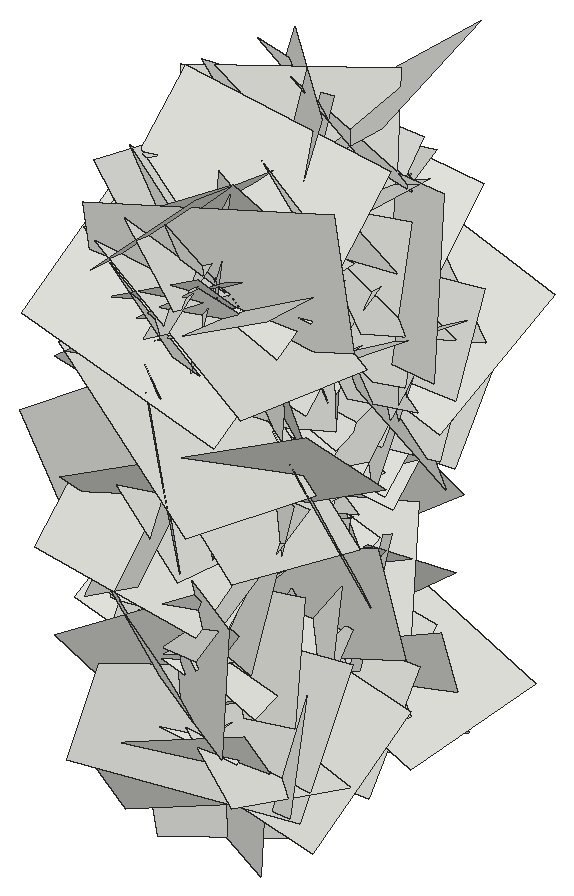
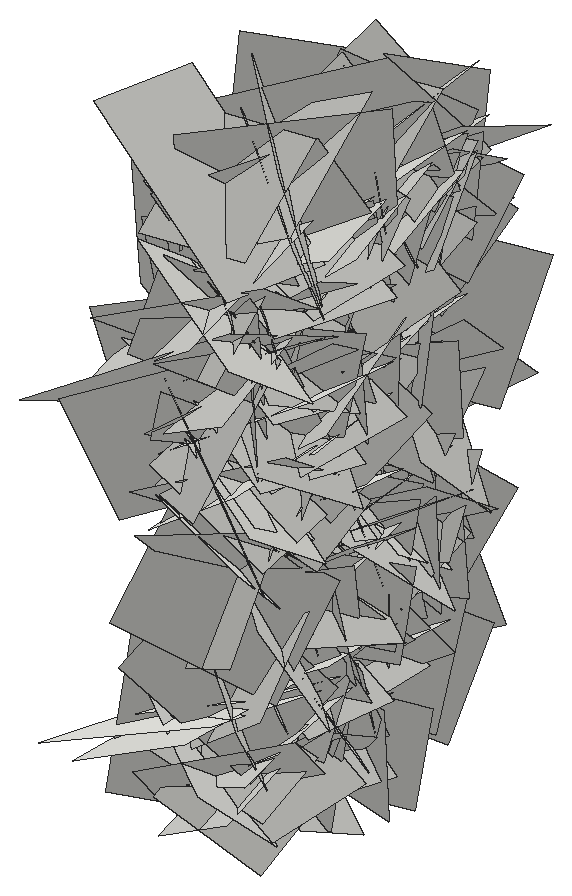
# SketchUp Ruby script. Lengths in inches.
U = 1.inch
M = Sketchup.active_model
def pt(a) = Geom::Point3d.new(a.map { |v| v * U })
def face(e, loops, mat)
  f = e.add_face(loops[0].map { |a| pt(a) })
  loops[1..].each { |l| e.add_face(l.map { |a| pt(a) }).erase! }
  f.material = f.back_material = mat if mat
  f
end
# faces: each face lists its corners as indices into pts; further lists are holes
def faces(e, pts, list, mat = nil) = list.each { |f| face(e, (f[0].is_a?(Array) ? f : [f]).map { |l| l.map { |i| pts[i] } }, mat) }
# xy, xz, yz: faces in a plane at the given z, y or x. An outline is a flat list of corners, or four numbers for a rectangle; further outlines are holes
def ring(l) = l.size == 4 ? [[l[0], l[1]], [l[2], l[1]], [l[2], l[3]], [l[0], l[3]]] : l.each_slice(2).to_a
def flat(e, list, mat, &to3) = list.each { |f| face(e, (f[0].is_a?(Array) ? f : [f]).map { |l| ring(l).map { |u, v| to3.(u, v) } }, mat) }
def xy(e, z, list, mat = nil) = flat(e, list, mat) { |x, y| [x, y, z] }
def xz(e, y, list, mat = nil) = flat(e, list, mat) { |x, z| [x, y, z] }
def yz(e, x, list, mat = nil) = flat(e, list, mat) { |y, z| [x, y, z] }
def lines(e, pts, list) = list.each { |a, b| e.add_line(pt(pts[a]), pt(pts[b])) }
# prism: a flat outline (further loops are holes) pulled along v
def prism(e, loops, v, mat = nil)
  f = face(e, loops, mat); d = Geom::Vector3d.new(v.map { |x| x * U })
  f.pushpull(f.normal.samedirection?(d) ? d.length : -d.length)
end
def box(e, o, s, mat = nil) = prism(e, [[o, [o[0] + s[0], o[1], o[2]], [o[0] + s[0], o[1] + s[1], o[2]], [o[0], o[1] + s[1], o[2]]]], [0, 0, s[2]], mat)
def at(x, y, z, deg = 0) = Geom::Transformation.translation(pt([x, y, z])) * Geom::Transformation.rotation(ORIGIN, Z_AXIS, deg.degrees)
def axes(o, x, y, z) = Geom::Transformation.new([*x, 0, *y, 0, *z, 0, *pt(o).to_a, 1])
def part(name) = M.definitions.add(name)
# library, detail: a bought-in or finely detailed component or shape, given as its bounding box
def library(name, o, s) = part(name).tap { |d| box(d.entities, o, s) }
def detail(e, o, s) = box(e.add_group.entities, o, s)
def put(e, d, t, mat = nil) = e.add_instance(d, t).tap { |i| i.material = mat if mat }
def group(e, t, mat = nil) = e.add_group.tap { |g| g.transformation = t; g.material = mat if mat }.entities
root = M.entities
c1 = part("Component\#6")
p = [[0.01,0,0],[0,3.24,4.54],[4.32,3.24,4.54],[4.33,0,0]]
faces(c1.entities,p,[[0,1,2,3]])
put(root,c1,axes([424.49,197.24,20.32],[-0.11105,0.4932,0.81979],[0.10012,0.82599,-0.48487],[-1.00916,0.02768,-0.13831]))
put(root,c1,axes([420.52,202.56,19.21],[0.06396,-0.26998,-0.58675],[-0.04641,-0.58965,0.26682],[0.68306,-0.01478,0.07307]))
put(root,c1,axes([420.52,199.64,2.06],[-0.21894,0.61345,0.59822],[0.01858,0.61825,-0.62794],[0.90807,0.13525,0.15708]))
put(root,c1,axes([424.49,196.07,8.125],[-0.08332,-0.69698,-0.457],[-0.10667,-0.44773,0.70016],[-0.87699,0.12068,-0.04174]))
put(root,c1,axes([420.52,190.79,19.57],[0.04866,0.55121,0.30162],[0.00575,0.30207,-0.55285],[0.66601,-0.04288,-0.01726]))
put(root,c1,axes([420.52,195.85,11.01],[-0.15114,0.73817,0.19544],[0.07767,0.21113,-0.74396],[0.80568,0.11812,0.10838]))
put(root,c1,axes([424.49,202.76,13.17],[0.11284,-1.03894,-0.17524],[-0.03066,-0.17895,1.04335],[-1.11641,-0.1001,-0.04636]))
put(root,c1,axes([424.49,189.31,11.46],[-0.01967,0.80876,0.77653],[0.21901,0.76581,-0.79265],[-1.16812,0.12996,-0.16169]))
put(root,c1,axes([420.52,193.57,4.75],[0.0218,0.6351,0.02763],[0.03876,0.02642,-0.63443],[0.67273,-0.0221,0.03566]))
put(root,c1,axes([424.49,199.68,18.17],[0.10811,0.81171,0.57509],[-0.11351,0.5837,-0.80488],[-1.04835,0.0205,0.14645]))
put(root,c1,axes([420.52,202.9,8.46],[-0.28421,-0.45126,-0.90988],[-0.10984,-0.92399,0.48879],[1.07096,-0.21452,-0.19133]))
put(root,c1,axes([420.52,193.91,15.9375],[0.03263,0.61645,-0.26034],[-0.02336,-0.25954,-0.61716],[0.70894,-0.03692,-0.00835]))
put(root,c1,axes([420.52,192.26,20.51],[-0.14395,0.6641,-0.62024],[-0.10915,-0.63433,-0.65665],[0.95701,0.02754,-0.16819]))
put(root,c1,axes([420.52,199.23,1.1],[-0.00098,-0.71414,-0.15761],[-0.04174,-0.15733,0.71311],[0.77408,-0.00939,0.03826]))
put(root,c1,axes([420.52,196.5625,6.92],[0.07674,-0.09799,-0.6482],[-0.03176,-0.65195,0.09521],[0.69417,-0.019,0.07601]))
put(root,c1,axes([420.52,198.91,12.75],[-0.15355,-0.10183,1.00426],[-0.21738,0.99636,0.07145],[1.04766,0.19182,0.16201]))
put(root,c1,axes([420.52,195.68,15.75],[0.06715,-0.51242,0.33521],[0.05381,0.34023,0.51051],[0.64683,0.02489,-0.07727]))
put(root,c1,axes([420.52,200.4375,8.06],[-0.17377,0.75884,-0.49804],[-0.05898,-0.51355,-0.76415],[0.96033,0.10576,-0.13705]))
put(root,c1,axes([420.52,199.6875,17.84],[0.07891,0.44569,0.39814],[0.07493,0.39183,-0.45185],[0.62903,-0.10259,0.00388]))
put(root,c1,axes([420.52,200.03,9.27],[-0.00412,-0.60297,0.30435],[0.07057,0.30253,0.60022],[0.71247,-0.03345,-0.05769]))
put(root,c1,axes([420.52,192.95,10.8],[0.02962,0.02518,0.78508],[-0.12702,0.77652,-0.02064],[0.82287,0.11896,-0.03145]))
put(root,c1,axes([424.49,199.37,10.67],[0.09558,-1.01864,0.46326],[0.13943,0.47118,1.01047],[-1.17795,-0.02688,0.1572]))
put(root,c1,axes([420.52,198.38,4.95],[-0.02223,0.32868,-0.55446],[0.17267,-0.53404,-0.32274],[0.66105,0.15055,0.06565]))
put(root,c1,axes([420.52,192.04,10.01],[-0.12172,0.5206,-0.6372],[0.01939,-0.6416,-0.52749],[0.87198,0.08694,-0.07722]))
put(root,c1,axes([420.52,202.51,19.98],[0.06792,0.48446,-0.5602],[-0.10116,-0.55221,-0.48846],[0.77852,-0.11402,-0.01459]))
put(root,c1,axes([424.49,195.86,16.68],[-0.06531,-0.43873,0.684],[-0.07025,0.68639,0.43429],[-0.8585,-0.02279,-0.08757]))
put(root,c1,axes([420.52,202.74,-0.14],[0.03158,-0.64507,0.25861],[0.01592,0.25938,0.64528],[0.73651,0.02205,-0.02503]))
put(root,c1,axes([424.49,192.22,20.81],[-0.00161,0.62306,-0.59539],[-0.0785,-0.59329,-0.62067],[-0.91013,0.05007,0.05459]))
put(root,c1,axes([420.52,197.35,3.52],[0.03443,0.41092,0.66217],[-0.08038,0.66126,-0.40665],[0.82215,0.04744,-0.06748]))
put(root,c1,axes([420.52,195.99,4.23],[-0.18601,0.0566,0.88651],[0.05201,0.90288,-0.04793],[0.94017,-0.03875,0.17804]))
put(root,c1,axes([424.49,198.67,11.97],[0.07539,0.76068,0.50866],[-0.0723,0.51318,-0.75791],[-0.96729,0.02092,0.0963]))
put(root,c1,axes([420.52,195.9375,9.16],[0.07841,0.69576,-0.29748],[-0.09095,-0.28926,-0.69787],[0.79692,-0.10147,-0.05038]))
put(root,c1,axes([424.49,195.4375,18.11],[-0.16874,-0.51977,-0.57708],[0.05885,-0.59519,0.52076],[-0.82114,0.06415,0.15591]))
put(root,c1,axes([424.49,196.17,12.88],[0.06274,0.02618,0.84664],[-0.15393,0.83645,-0.01571],[-0.88457,-0.1437,0.06278]))
put(root,c1,axes([424.49,193.46,10.77],[-0.10152,0.90556,-0.18731],[0.17799,-0.16815,-0.89879],[-0.96391,-0.12642,-0.14624]))
put(root,c1,axes([420.52,200.82,0.59],[0.02153,-0.73416,-0.35765],[-0.0933,-0.35764,0.72915],[0.8606,-0.02041,0.08799]))
put(root,c1,axes([424.49,195.73,16.63],[0.01219,-0.78698,0.32297],[-0.05977,0.32158,0.78561],[-0.89973,-0.03203,-0.04781]))
put(root,c1,axes([424.49,196.375,20.79],[0.12547,0.87042,-0.10702],[-0.18806,-0.08199,-0.86307],[-0.91037,0.1369,0.16354]))
put(root,c1,axes([424.49,200.05,13.66],[-0.07814,0.81604,-0.08962],[0.02759,-0.08761,-0.81916],[-0.86976,-0.0761,-0.01794]))
put(root,c1,axes([424.49,198.3125,4.47],[0.08144,0.93817,-0.09306],[0.01009,-0.09413,-0.94116],[-0.99929,0.07551,-0.01709]))
put(root,c1,axes([424.49,200.41,3.58],[0.05776,-0.87144,-0.04483],[-0.06577,-0.04867,0.87073],[-0.92261,-0.05109,-0.06488]))
put(root,c1,axes([424.49,195.95,14.86],[0.17446,0.9838,0.62037],[0.19333,0.59697,-0.99508],[-1.2176,0.23574,-0.06911]))
put(root,c1,axes([424.49,194.43,21.03],[0.18864,1.08922,-0.2367],[0.12278,-0.25647,-1.09312],[-1.17512,0.14806,-0.15221]))
put(root,c1,axes([420.52,200.69,6.875],[-0.16125,-0.91938,-0.30199],[-0.04119,-0.29965,0.93182],[1.02494,-0.15668,-0.01006]))
put(root,c1,axes([424.49,193.09,19.46],[-0.07295,0.25641,0.83596],[0.12348,0.83376,-0.24615],[-0.9186,0.09171,-0.09948]))
put(root,c1,axes([424.49,196.25,20.97],[-0.03433,0.46285,-0.75346],[0.09275,-0.74858,-0.46362],[-0.93272,-0.09148,-0.01837]))
put(root,c1,axes([420.52,193.9,23.36],[0.05376,0.55183,-0.55937],[-0.04326,-0.55793,-0.55411],[0.83178,-0.06469,0.00734]))
put(root,c1,axes([424.49,193.92,18.08],[0.13809,0.41624,-1.10581],[0.27382,-1.09563,-0.38198],[-1.22215,-0.19844,-0.21052]))
put(root,c1,axes([424.49,202.38,16.09],[0.07402,-0.92988,-0.45649],[0.17154,-0.44211,0.92536],[-1.08456,-0.13339,0.1152]))
put(root,c1,axes([420.52,201.99,11.3125],[-0.07595,0.62186,-0.76254],[-0.14567,-0.76339,-0.60964],[1.03278,-0.06194,-0.14206]))
put(root,c1,axes([420.52,202.11,15.27],[0.00741,-0.76642,-0.19435],[0.02033,-0.19414,0.76626],[0.83787,0.01149,-0.01688]))
put(root,c1,axes([424.49,195.27,-1.16],[0.10176,-0.07093,0.82892],[-0.16666,0.81783,0.08819],[-0.86597,-0.16573,0.08043]))
put(root,c1,axes([424.49,196.11,19.5625],[0.1708,0.27531,1.11719],[0.21419,1.10379,-0.30115],[-1.2007,0.23607,0.1052]))
put(root,c1,axes([420.52,200.46,4.14],[0.03987,0.66432,-0.22968],[0.12809,-0.2327,-0.65325],[0.73398,0.00452,0.12648]))
put(root,c1,axes([424.49,200.85,9.74],[-0.02518,0.49854,0.49521],[-0.19267,0.47427,-0.48618],[-0.7195,-0.14445,0.11286]))
put(root,c1,axes([420.52,192.1875,23.6],[0.04344,0.89705,-0.17333],[-0.1764,-0.16328,-0.88435],[0.95226,-0.07116,-0.15591]))
put(root,c1,axes([424.49,192.1875,23.6],[-0.04344,0.89705,-0.17333],[0.1764,-0.16328,-0.88435],[-0.95226,-0.07116,-0.15591]))
put(root,c1,axes([420.52,200.85,9.74],[0.02518,0.49854,0.49521],[0.19267,0.47427,-0.48618],[0.7195,-0.14445,0.11286]))
put(root,c1,axes([424.49,200.46,4.14],[-0.03987,0.66432,-0.22968],[-0.12809,-0.2327,-0.65325],[-0.73398,0.00452,0.12648]))
put(root,c1,axes([420.52,196.11,19.5625],[-0.1708,0.27531,1.11719],[-0.21419,1.10379,-0.30115],[1.2007,0.23607,0.1052]))
put(root,c1,axes([420.52,195.27,-1.16],[-0.10176,-0.07093,0.82892],[0.16666,0.81783,0.08819],[0.86597,-0.16573,0.08043]))
put(root,c1,axes([424.49,202.11,15.27],[-0.00741,-0.76642,-0.19435],[-0.02033,-0.19414,0.76626],[-0.83787,0.01149,-0.01688]))
put(root,c1,axes([424.49,201.99,11.3125],[0.07595,0.62186,-0.76254],[0.14567,-0.76339,-0.60964],[-1.03278,-0.06194,-0.14206]))
put(root,c1,axes([420.52,202.38,16.09],[-0.07402,-0.92988,-0.45649],[-0.17154,-0.44211,0.92536],[1.08456,-0.13339,0.1152]))
put(root,c1,axes([420.52,193.92,18.08],[-0.13809,0.41624,-1.10581],[-0.27382,-1.09563,-0.38198],[1.22215,-0.19844,-0.21052]))
put(root,c1,axes([424.49,193.9,23.36],[-0.05376,0.55183,-0.55937],[0.04326,-0.55793,-0.55411],[-0.83178,-0.06469,0.00734]))
put(root,c1,axes([420.52,196.25,20.97],[0.03433,0.46285,-0.75346],[-0.09275,-0.74858,-0.46362],[0.93272,-0.09148,-0.01837]))
put(root,c1,axes([420.52,193.09,19.46],[0.07295,0.25641,0.83596],[-0.12348,0.83376,-0.24615],[0.9186,0.09171,-0.09948]))
put(root,c1,axes([424.49,200.69,6.875],[0.16125,-0.91938,-0.30199],[0.04119,-0.29965,0.93182],[-1.02494,-0.15668,-0.01006]))
put(root,c1,axes([420.52,194.43,21.03],[-0.18864,1.08922,-0.2367],[-0.12278,-0.25647,-1.09312],[1.17512,0.14806,-0.15221]))
put(root,c1,axes([420.52,195.95,14.86],[-0.17446,0.9838,0.62037],[-0.19333,0.59697,-0.99508],[1.2176,0.23574,-0.06911]))
put(root,c1,axes([420.52,200.41,3.58],[-0.05776,-0.87144,-0.04483],[0.06577,-0.04867,0.87073],[0.92261,-0.05109,-0.06488]))
put(root,c1,axes([420.52,198.3125,4.47],[-0.08144,0.93817,-0.09306],[-0.01009,-0.09413,-0.94116],[0.99929,0.07551,-0.01709]))
put(root,c1,axes([420.52,200.05,13.66],[0.07814,0.81604,-0.08962],[-0.02759,-0.08761,-0.81916],[0.86976,-0.0761,-0.01794]))
put(root,c1,axes([420.52,196.375,20.79],[-0.12547,0.87042,-0.10702],[0.18806,-0.08199,-0.86307],[0.91037,0.1369,0.16354]))
put(root,c1,axes([420.52,195.73,16.63],[-0.01219,-0.78698,0.32297],[0.05977,0.32158,0.78561],[0.89973,-0.03203,-0.04781]))
put(root,c1,axes([424.49,200.82,0.59],[-0.02153,-0.73416,-0.35765],[0.0933,-0.35764,0.72915],[-0.8606,-0.02041,0.08799]))
put(root,c1,axes([420.52,193.46,10.77],[0.10152,0.90556,-0.18731],[-0.17799,-0.16815,-0.89879],[0.96391,-0.12642,-0.14624]))
put(root,c1,axes([420.52,196.17,12.88],[-0.06274,0.02618,0.84664],[0.15393,0.83645,-0.01571],[0.88457,-0.1437,0.06278]))
put(root,c1,axes([420.52,195.4375,18.11],[0.16874,-0.51977,-0.57708],[-0.05885,-0.59519,0.52076],[0.82114,0.06415,0.15591]))
put(root,c1,axes([424.49,195.9375,9.16],[-0.07841,0.69576,-0.29748],[0.09095,-0.28926,-0.69787],[-0.79692,-0.10147,-0.05038]))
put(root,c1,axes([420.52,198.67,11.97],[-0.07539,0.76068,0.50866],[0.0723,0.51318,-0.75791],[0.96729,0.02092,0.0963]))
put(root,c1,axes([424.49,195.99,4.23],[0.18601,0.0566,0.88651],[-0.05201,0.90288,-0.04793],[-0.94017,-0.03875,0.17804]))
put(root,c1,axes([424.49,197.35,3.52],[-0.03443,0.41092,0.66217],[0.08038,0.66126,-0.40665],[-0.82215,0.04744,-0.06748]))
put(root,c1,axes([420.52,192.22,20.81],[0.00161,0.62306,-0.59539],[0.0785,-0.59329,-0.62067],[0.91013,0.05007,0.05459]))
put(root,c1,axes([424.49,202.74,-0.14],[-0.03158,-0.64507,0.25861],[-0.01592,0.25938,0.64528],[-0.73651,0.02205,-0.02503]))
put(root,c1,axes([420.52,195.86,16.68],[0.06531,-0.43873,0.684],[0.07025,0.68639,0.43429],[0.8585,-0.02279,-0.08757]))
put(root,c1,axes([424.49,202.51,19.98],[-0.06792,0.48446,-0.5602],[0.10116,-0.55221,-0.48846],[-0.77852,-0.11402,-0.01459]))
put(root,c1,axes([424.49,192.04,10.01],[0.12172,0.5206,-0.6372],[-0.01939,-0.6416,-0.52749],[-0.87198,0.08694,-0.07722]))
put(root,c1,axes([424.49,198.38,4.95],[0.02223,0.32868,-0.55446],[-0.17267,-0.53404,-0.32274],[-0.66105,0.15055,0.06565]))
put(root,c1,axes([420.52,199.37,10.67],[-0.09558,-1.01864,0.46326],[-0.13943,0.47118,1.01047],[1.17795,-0.02688,0.1572]))
put(root,c1,axes([424.49,192.95,10.8],[-0.02962,0.02518,0.78508],[0.12702,0.77652,-0.02064],[-0.82287,0.11896,-0.03145]))
put(root,c1,axes([424.49,200.03,9.27],[0.00412,-0.60297,0.30435],[-0.07057,0.30253,0.60022],[-0.71247,-0.03345,-0.05769]))
put(root,c1,axes([424.49,199.6875,17.84],[-0.07891,0.44569,0.39814],[-0.07493,0.39183,-0.45185],[-0.62903,-0.10259,0.00388]))
put(root,c1,axes([424.49,200.4375,8.06],[0.17377,0.75884,-0.49804],[0.05898,-0.51355,-0.76415],[-0.96033,0.10576,-0.13705]))
put(root,c1,axes([424.49,195.68,15.75],[-0.06715,-0.51242,0.33521],[-0.05381,0.34023,0.51051],[-0.64683,0.02489,-0.07727]))
put(root,c1,axes([424.49,198.91,12.75],[0.15355,-0.10183,1.00426],[0.21738,0.99636,0.07145],[-1.04766,0.19182,0.16201]))
put(root,c1,axes([424.49,196.5625,6.92],[-0.07674,-0.09799,-0.6482],[0.03176,-0.65195,0.09521],[-0.69417,-0.019,0.07601]))
put(root,c1,axes([424.49,199.23,1.1],[0.00098,-0.71414,-0.15761],[0.04174,-0.15733,0.71311],[-0.77408,-0.00939,0.03826]))
put(root,c1,axes([424.49,192.26,20.51],[0.14395,0.6641,-0.62024],[0.10915,-0.63433,-0.65665],[-0.95701,0.02754,-0.16819]))
put(root,c1,axes([424.49,193.91,15.9375],[-0.03263,0.61645,-0.26034],[0.02336,-0.25954,-0.61716],[-0.70894,-0.03692,-0.00835]))
put(root,c1,axes([424.49,202.9,8.46],[0.28421,-0.45126,-0.90988],[0.10984,-0.92399,0.48879],[-1.07096,-0.21452,-0.19133]))
put(root,c1,axes([420.52,199.68,18.17],[-0.10811,0.81171,0.57509],[0.11351,0.5837,-0.80488],[1.04835,0.0205,0.14645]))
put(root,c1,axes([424.49,193.57,4.75],[-0.0218,0.6351,0.02763],[-0.03876,0.02642,-0.63443],[-0.67273,-0.0221,0.03566]))
put(root,c1,axes([420.52,189.31,11.46],[0.01967,0.80876,0.77653],[-0.21901,0.76581,-0.79265],[1.16812,0.12996,-0.16169]))
put(root,c1,axes([420.52,202.76,13.17],[-0.11284,-1.03894,-0.17524],[0.03066,-0.17895,1.04335],[1.11641,-0.1001,-0.04636]))
put(root,c1,axes([424.49,195.85,11.01],[0.15114,0.73817,0.19544],[-0.07767,0.21113,-0.74396],[-0.80568,0.11812,0.10838]))
put(root,c1,axes([424.49,190.79,19.57],[-0.04866,0.55121,0.30162],[-0.00575,0.30207,-0.55285],[-0.66601,-0.04288,-0.01726]))
put(root,c1,axes([420.52,196.07,8.125],[0.08332,-0.69698,-0.457],[0.10667,-0.44773,0.70016],[0.87699,0.12068,-0.04174]))
put(root,c1,axes([424.49,199.64,2.06],[0.21894,0.61345,0.59822],[-0.01858,0.61825,-0.62794],[-0.90807,0.13525,0.15708]))
put(root,c1,axes([424.49,202.56,19.21],[-0.06396,-0.26998,-0.58675],[0.04641,-0.58965,0.26682],[-0.68306,-0.01478,0.07307]))
put(root,c1,axes([420.52,197.24,20.32],[0.11105,0.4932,0.81979],[-0.10012,0.82599,-0.48487],[1.00916,0.02768,-0.13831]))
put(root,c1,axes([420.52,196.19,13.89],[-0.03711,0.95345,-0.08325],[0.1071,-0.07916,-0.94908],[1.00884,0.04348,0.09769]))
put(root,c1,axes([424.49,198.53,13.8],[0.10676,-0.41647,0.70694],[0.09382,0.7136,0.40779],[-0.86465,0.02601,0.13154]))
put(root,c1,axes([424.49,201.03,8.02],[0.03451,-0.61291,-0.20918],[-0.0475,-0.21108,0.61149],[-0.68484,-0.01625,-0.05296]))
put(root,c1,axes([424.49,199.53,17.66],[0.07108,0.22718,0.77768],[0.14032,0.76678,-0.23541],[-0.84726,0.14605,0.02626]))
put(root,c1,axes([424.49,196.1,5.28],[0.08762,-0.56519,-0.39893],[-0.0287,-0.4041,0.56691],[-0.73275,-0.05175,-0.06991]))
put(root,c1,axes([420.52,192.44,8.79],[-0.05887,1.04295,0.25043],[0.00297,0.2509,-1.04431],[1.13694,0.05335,0.0157]))
put(root,c1,axes([420.52,193.71,0.46],[0.00413,-0.52236,0.7551],[0.18121,0.74232,0.51263],[0.95624,-0.13842,-0.10041]))
put(root,c1,axes([420.52,195.28,4.79],[0.03702,0.87634,0.85063],[-0.28559,0.83554,-0.84973],[1.26267,0.16329,-0.21713]))
put(root,c1,axes([420.52,203.91,5.3125],[0.18463,-0.58129,-0.78091],[-0.13848,-0.80009,0.56643],[1.02258,-0.00339,0.2177]))
put(root,c1,axes([420.52,198.93,5.125],[0.08676,0.85287,0.14934],[0.16568,0.13299,-0.84515],[0.90272,-0.10637,0.14076]))
put(root,c1,axes([420.52,198.84,9.75],[-0.24721,-0.9594,-0.88495],[-0.06038,-0.89063,0.98057],[1.38221,-0.2105,-0.11544]))
put(root,c1,axes([420.52,202.1,18.26],[-0.1919,-1.13475,-0.09678],[0.16378,-0.12156,1.13628],[1.19604,-0.16542,-0.17113]))
put(root,c1,axes([424.49,194.11,10.49],[0.01019,-0.66626,0.06574],[0.1187,0.06642,0.65679],[-0.69967,0.00157,0.11238]))
put(root,c1,axes([420.52,200.51,5.45],[-0.07717,-0.59417,-0.91785],[0.09928,-0.91989,0.58806],[1.15472,0.03938,-0.1119]))
put(root,c1,axes([420.52,205.24,14.9],[-0.1168,-0.46047,-1.13614],[-0.0362,-1.13913,0.465],[1.29896,-0.07315,-0.0892]))
put(root,c1,axes([420.52,194.25,1.05],[0.1707,-0.55728,0.79671],[-0.04122,0.80323,0.5697],[1.02978,0.12452,-0.10926]))
put(root,c1,axes([420.52,194.35,10.5],[-0.1187,0.07765,-1.12146],[0.14385,-1.11784,-0.09095],[1.18288,0.14373,-0.10148]))
put(root,c1,axes([420.52,188.68,19.83],[-0.08458,1.11358,0.50301],[-0.01593,0.50315,-1.11627],[1.29513,0.07891,0.01912]))
put(root,c1,axes([420.52,197.36,24.8],[-0.09794,1.0389,-0.68546],[-0.01654,-0.68826,-1.04104],[1.31923,0.0685,-0.06394]))
put(root,c1,axes([424.49,199.74,12.37],[0.13977,-0.41949,-0.41774],[-0.0557,-0.43458,0.41982],[-0.62506,-0.05508,-0.13082]))
put(root,c1,axes([424.49,199.42,15.6],[0.03605,-0.49998,-0.38134],[0.14474,-0.36691,0.49324],[-0.65063,-0.10932,0.0886]))
put(root,c1,axes([420.52,200.08,24.34],[0.03463,0.75517,-0.67877],[0.20748,-0.67107,-0.73718],[1.05612,0.10708,0.16708]))
put(root,c1,axes([420.52,199.09,16.39],[0.13116,-1.14374,0.05938],[-0.13174,0.04596,1.1443],[1.20683,0.12933,0.11846]))
put(root,c1,axes([420.52,192.66,5.0625],[0.03803,0.06475,1.02957],[0.25075,1.00223,-0.07127],[1.06436,-0.23842,-0.02]))
put(root,c1,axes([420.52,196.53,2.03],[0.14871,0.38131,0.94323],[0.09041,0.94439,-0.39446],[1.07463,-0.13222,-0.09734]))
put(root,c1,axes([420.52,200.2,14.91],[0.20407,-0.96139,-0.18597],[0.07393,-0.17559,0.97991],[1.03533,0.20204,-0.03331]))
put(root,c1,axes([420.52,198.375,11.05],[-0.00636,-0.47599,-1.14741],[-0.03555,-1.14695,0.47597],[1.31628,-0.03327,0.00731]))
put(root,c1,axes([420.52,202.25,12.93],[-0.19135,-1.27912,0.12446],[0.2118,0.09622,1.27869],[1.34571,-0.19703,-0.18355]))
put(root,c1,axes([420.52,197.86,18.23],[0.19608,0.2602,-1.0463],[-0.01915,-1.06069,-0.26697],[1.14269,-0.06243,0.17507]))
put(root,c1,axes([420.52,197.84,4.84],[0.11369,-0.36766,-0.96616],[0.19069,-0.94989,0.38144],[1.07906,0.2066,0.03439]))
put(root,c1,axes([420.52,200.375,7.61],[0.26418,-0.51362,-0.84712],[0.05211,-0.86603,0.53955],[1.04881,0.1724,0.18657]))
put(root,c1,axes([420.52,203.04,12.11],[0.14841,-0.94408,-0.5752],[0.05434,-0.57362,0.95398],[1.17058,0.14632,0.02864]))
put(root,c1,axes([420.52,199.56,18.73],[0.07364,1.07871,-0.62029],[-0.05176,-0.61841,-1.08091],[1.31797,-0.08456,-0.00779]))
put(root,c1,axes([420.52,204.42,20.53],[0.1154,-1.25003,-0.28156],[-0.14973,-0.29256,1.24425],[1.34995,0.07441,0.16208]))
put(root,c1,axes([420.52,195.93,15.54],[0.04965,0.25406,1.2028],[0.02984,1.20314,-0.25523],[1.30276,-0.03724,-0.03999]))
put(root,c1,axes([420.52,198.85,12.57],[0.15345,0.48368,1.12599],[-0.09378,1.13498,-0.47617],[1.29562,0.02486,-0.16783]))
put(root,c1,axes([420.52,200.7,5.85],[0.20906,1.0682,-0.14016],[0.07965,-0.15578,-1.08152],[1.13921,-0.18514,0.10133]))
put(root,c1,axes([420.52,194.09,6.34],[0.25898,1.07168,-0.21064],[-0.01285,-0.21318,-1.09862],[1.15764,-0.24212,0.03493]))
put(root,c1,axes([420.52,192.7,21.39],[0.08893,0.79245,0.9015],[0.06254,0.89988,-0.79652],[1.27076,-0.09974,-0.02389]))
put(root,c1,axes([420.52,199.38,-0.0625],[0.15183,-0.50198,1.07326],[0.00307,1.08122,0.50532],[1.25594,0.05804,-0.13098]))
put(root,c1,axes([420.52,192.73,15.73],[0.12897,1.2724,-0.23633],[-0.08155,-0.22984,-1.27707],[1.36939,-0.13352,-0.05379]))
put(root,c1,axes([420.52,200.21,21.54],[0.14018,1.21556,-0.55877],[-0.14242,-0.54659,-1.22085],[1.41094,-0.17594,-0.06772]))
put(root,c1,axes([420.52,190.45,18.05],[0.16537,1.24759,-0.14593],[-0.05265,-0.14081,-1.25691],[1.33042,-0.16065,-0.0316]))
put(root,c1,axes([420.52,190.86,3.39],[0.21383,0.32739,1.20741],[-0.09698,1.22359,-0.31649],[1.32251,0.03679,-0.21843]))
put(root,c1,axes([420.52,195.52,16.87],[0.17814,-1.09516,0.21581],[0.19304,0.24222,1.08736],[1.16734,0.12707,-0.21275]))
put(root,c1,axes([420.52,201.79,17.38],[0.19939,0.73728,-1.06028],[-0.09629,-1.06126,-0.75408],[1.36551,-0.18249,0.10164]))
put(root,c1,axes([420.52,196.26,4.8],[0.10051,-0.43998,1.12809],[0.21352,1.12151,0.42048],[1.26562,-0.15427,-0.16053]))
put(root,c1,axes([420.52,191.67,21.5],[0.0579,1.33618,-0.15223],[0.05318,-0.15428,-1.33612],[1.42453,-0.04855,0.05606]))
put(root,c1,axes([420.52,198.6875,16.83],[0.02201,1.26014,0.56955],[0.0456,0.56875,-1.25994],[1.46513,-0.03663,0.03065]))
put(root,c1,axes([420.52,196.95,13.22],[0.12152,0.35472,1.26895],[0.01769,1.27325,-0.35743],[1.39654,-0.047,-0.10589]))
put(root,c1,axes([420.52,197.84,15.77],[0.08558,0.66637,-1.22765],[0.01617,-1.23004,-0.66667],[1.48057,-0.02508,0.07824]))
put(root,c1,axes([420.52,193.34,3.5],[0.3285,0.68164,0.95344],[0.04901,0.97833,-0.71446],[1.2414,-0.219,-0.22409]))
put(root,c1,axes([420.52,192.59,17.15],[0.08597,-0.32374,1.28455],[0.18245,1.27862,0.31138],[1.3923,-0.14756,-0.12012]))
put(root,c1,axes([420.52,199.09,4.9],[0.11121,1.25407,0.182],[0.25083,0.16003,-1.23904],[1.31962,-0.1361,0.22018]))
put(root,c1,axes([420.52,194.4,9.86],[0.11876,-1.04596,0.91618],[0.1474,0.92297,1.03671],[1.46651,-0.00807,-0.1784]))
put(root,c1,axes([420.52,202.95,19.72],[0.19445,-0.3512,-1.29554],[0.25274,-1.27827,0.38028],[1.40021,0.2795,0.11127]))
